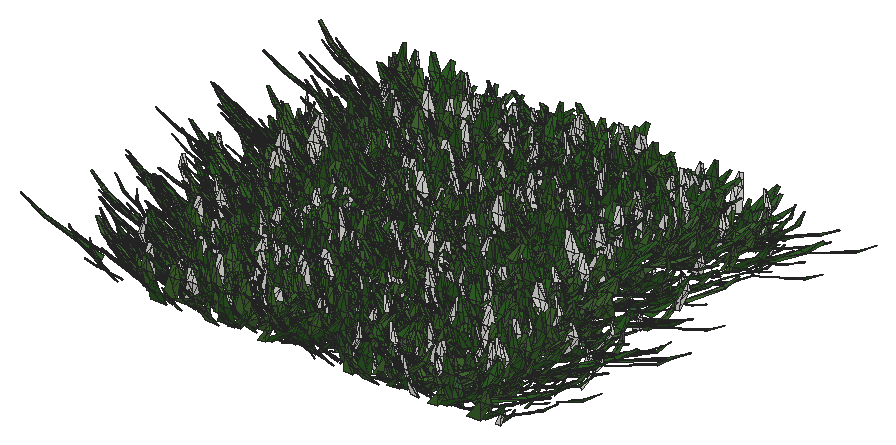
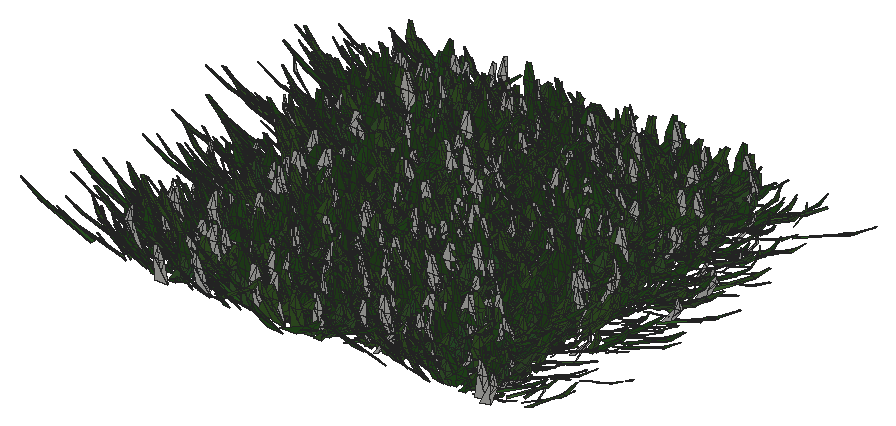
# SketchUp Ruby script. Lengths in inches.
U = 1.inch
M = Sketchup.active_model
def pt(a) = Geom::Point3d.new(a.map { |v| v * U })
def face(e, loops, mat)
  f = e.add_face(loops[0].map { |a| pt(a) })
  loops[1..].each { |l| e.add_face(l.map { |a| pt(a) }).erase! }
  f.material = f.back_material = mat if mat
  f
end
# faces: each face lists its corners as indices into pts; further lists are holes
def faces(e, pts, list, mat = nil) = list.each { |f| face(e, (f[0].is_a?(Array) ? f : [f]).map { |l| l.map { |i| pts[i] } }, mat) }
# xy, xz, yz: faces in a plane at the given z, y or x. An outline is a flat list of corners, or four numbers for a rectangle; further outlines are holes
def ring(l) = l.size == 4 ? [[l[0], l[1]], [l[2], l[1]], [l[2], l[3]], [l[0], l[3]]] : l.each_slice(2).to_a
def flat(e, list, mat, &to3) = list.each { |f| face(e, (f[0].is_a?(Array) ? f : [f]).map { |l| ring(l).map { |u, v| to3.(u, v) } }, mat) }
def xy(e, z, list, mat = nil) = flat(e, list, mat) { |x, y| [x, y, z] }
def xz(e, y, list, mat = nil) = flat(e, list, mat) { |x, z| [x, y, z] }
def yz(e, x, list, mat = nil) = flat(e, list, mat) { |y, z| [x, y, z] }
def lines(e, pts, list) = list.each { |a, b| e.add_line(pt(pts[a]), pt(pts[b])) }
# prism: a flat outline (further loops are holes) pulled along v
def prism(e, loops, v, mat = nil)
  f = face(e, loops, mat); d = Geom::Vector3d.new(v.map { |x| x * U })
  f.pushpull(f.normal.samedirection?(d) ? d.length : -d.length)
end
def box(e, o, s, mat = nil) = prism(e, [[o, [o[0] + s[0], o[1], o[2]], [o[0] + s[0], o[1] + s[1], o[2]], [o[0], o[1] + s[1], o[2]]]], [0, 0, s[2]], mat)
def at(x, y, z, deg = 0) = Geom::Transformation.translation(pt([x, y, z])) * Geom::Transformation.rotation(ORIGIN, Z_AXIS, deg.degrees)
def axes(o, x, y, z) = Geom::Transformation.new([*x, 0, *y, 0, *z, 0, *pt(o).to_a, 1])
def part(name) = M.definitions.add(name)
# library, detail: a bought-in or finely detailed component or shape, given as its bounding box
def library(name, o, s) = part(name).tap { |d| box(d.entities, o, s) }
def detail(e, o, s) = box(e.add_group.entities, o, s)
def put(e, d, t, mat = nil) = e.add_instance(d, t).tap { |i| i.material = mat if mat }
def group(e, t, mat = nil) = e.add_group.tap { |g| g.transformation = t; g.material = mat if mat }.entities
root = M.entities
M.materials.add("Material10").color = [48, 100, 38]
M.materials.add("Material3").color = [68, 110, 58]
M.materials.add("Material4").color = [48, 90, 38]
M.materials.add("Material5").color = [68, 110, 48]
M.materials.add("Material6").color = [48, 90, 48]
M.materials.add("Material7").color = [58, 110, 58]
M.materials.add("Material8").color = [58, 90, 38]
M.materials.add("Material9").color = [68, 100, 58]
c1 = part("grass00")
p = [[-0.6875,0.15,0],[-0.56,0.08,5.52],[-0.04,0.03,2.76],[0.48,-0.02,0],[0.35,-0.02,5.52],[-0.1,-0.14,5.52],
  [-0.12,0.65,8.37],[-0.42,0.65,8.37]]
faces(c1.entities,p,[[0,1,2,3],[3,2,4],[1,5,2],[5,4,2],[1,6,5],[4,5,6],[7,6,1]])
c2 = part("Group16\#1")
put(c2.entities,c1,axes([1.44,-0.61,-0.01],[0.05352,0.12609,0],[-0.10704,0.04543,0.07239],[0.06664,-0.02828,0.11628]),"Material6")
put(c2.entities,c1,axes([0.76,-0.15,-0.01],[0.04676,0.24062,0],[-0.23162,0.04501,0.06642],[0.0652,-0.01267,0.23595]),"Material3")
put(c2.entities,c1,axes([0.79,0.01,-0.01],[-0.00606,0.34651,0],[-0.34381,-0.00602,0.0432],[0.04319,0.00076,0.34386]))
put(c2.entities,c1,axes([1,0.23,-0.01],[-0.07192,0.31144,0],[-0.28722,-0.06632,0.1236],[0.12043,0.02781,0.29478]),"Material5")
put(c2.entities,c1,axes([1.66,0.77,-0.01],[-0.13828,0.29651,0],[-0.21551,-0.1005,0.22471],[0.20365,0.09498,0.23779]),"Material10")
put(c2.entities,c1,axes([0.6875,0.52,-0.01],[-0.18126,0.24051,0],[-0.22746,-0.17142,0.09788],[0.07817,0.05891,0.28481]),"Material5")
put(c2.entities,c1,axes([0.68,0.78,-0.01],[-0.215,0.18688,0],[-0.12385,-0.14248,0.21334],[0.13995,0.16101,0.18878]),"Material3")
put(c2.entities,c1,axes([0.56,1,-0.01],[-0.13756,0.07624,0],[-0.06159,-0.11112,0.0927],[0.04494,0.08108,0.12705]),"Material5")
put(c2.entities,c1,axes([0.2,0.64,-0.01],[-0.23729,0.07254,0],[-0.05711,-0.18681,0.153],[0.04473,0.14632,0.19535]),"Material10")
put(c2.entities,c1,axes([0.0625,0.72,-0.01],[-0.28874,0.02525,0],[-0.02179,-0.24916,0.14647],[0.01276,0.14591,0.25012]),"Material3")
put(c2.entities,c1,axes([-0.08,0.62,-0.01],[-0.34089,-0.04187,0],[0.03255,-0.26504,0.216],[-0.02633,0.21439,0.26703]),"Material10")
put(c2.entities,c1,axes([-0.34,0.98,-0.01],[-0.14314,-0.0493,0],[0.04397,-0.12769,0.06843],[-0.02228,0.0647,0.13505]),"Material10")
put(c2.entities,c1,axes([-0.87,1.45,-0.01],[-0.23488,-0.14114,0],[0.13761,-0.22901,0.06087],[-0.03135,0.05217,0.26717]))
put(c2.entities,c1,axes([-0.72,0.77,-0.01],[-0.14208,-0.13251,0],[0.07209,-0.0773,0.16301],[-0.11118,0.11922,0.1057]),"Material10")
put(c2.entities,c1,axes([-0.62,0.43,-0.01],[-0.14845,-0.21203,0],[0.18654,-0.13061,0.12304],[-0.10079,0.07057,0.22772]),"Material3")
put(c2.entities,c1,axes([-0.68,0.29,-0.01],[-0.13639,-0.32136,0],[0.31723,-0.13464,0.05579],[-0.05136,0.0218,0.34462]),"Material4")
put(c2.entities,c1,axes([-0.64,0.125,-0.01],[-0.0458,-0.23569,0],[0.22124,-0.043,0.08276],[-0.08124,0.01579,0.22538]),"Material7")
put(c2.entities,c1,axes([-1.6,-0.03,-0.01],[0.00576,-0.32897,0],[0.27526,0.00482,0.18018],[-0.18015,-0.00315,0.2753]),"Material5")
put(c2.entities,c1,axes([-1.36,-0.31,-0.01],[0.05718,-0.24765,0],[0.18172,0.04196,0.17267],[-0.16825,-0.03885,0.1865]),"Material10")
put(c2.entities,c1,axes([-1.54,-0.72,-0.01],[0.06537,-0.14017,0],[0.13555,0.06321,0.03939],[-0.0357,-0.01665,0.14956]))
put(c2.entities,c1,axes([-1.19,-0.9,-0.01],[0.09597,-0.12735,0],[0.11214,0.08451,0.07557],[-0.06035,-0.04548,0.14042]),"Material9")
put(c2.entities,c1,axes([-0.47,-0.54,-0.01],[0.11588,-0.10072,0],[0.0618,0.0711,0.12124],[-0.07953,-0.0915,0.0942]))
put(c2.entities,c1,axes([-0.47,-0.84,-0.01],[0.11927,-0.0661,0],[0.06603,0.11913,0.00646],[-0.00313,-0.00565,0.13621]),"Material5")
put(c2.entities,c1,axes([-0.38,-1.24,-0.01],[0.28037,-0.08571,0],[0.0618,0.20215,0.20315],[-0.05939,-0.19428,0.21139]),"Material9")
put(c2.entities,c1,axes([-0.06,-0.66,-0.01],[0.22719,-0.01987,0],[0.01247,0.14255,0.17758],[-0.01547,-0.17691,0.1431]),"Material8")
put(c2.entities,c1,axes([0.11,-0.89,-0.01],[0.14882,0.01828,0],[-0.01058,0.08611,0.12229],[0.01491,-0.12138,0.08676]),"Material6")
put(c2.entities,c1,axes([0.25,-0.72,-0.01],[0.20481,0.07053,0],[-0.06206,0.18022,0.10291],[0.03351,-0.0973,0.1906]),"Material6")
put(c2.entities,c1,axes([0.85,-1.42,-0.01],[0.16481,0.09904,0],[-0.09472,0.15762,0.05616],[0.02893,-0.04814,0.18389]),"Material5")
put(c2.entities,c1,axes([1.01,-1.09,-0.01],[0.21858,0.20385,0],[-0.17495,0.1876,0.15339],[0.10462,-0.11218,0.25652]),"Material10")
put(c2.entities,c1,axes([1.01,-0.71,-0.01],[0.08733,0.12473,0],[-0.06445,0.04512,0.13037],[0.1068,-0.07477,0.07867]),"Material6")
c3 = part("Group15\#1")
put(c3.entities,c2,at(0,0,0))
c4 = part("3darcstudiotree_grass00\#1")
put(c4.entities,c3,at(0,0,0))
put(root,c4,axes([260.58,70.62,7.6],[-3.85189,-0.43073,0],[1.56903,-0.87695,-0.00732],[0.02092,-0.01169,1.68082]))
put(root,c4,axes([260.53,52.63,7.6],[-1.50152,-0.9142,0],[4.09435,-0.4203,-0.04381],[0.2556,-0.02624,1.74465]))
put(root,c4,axes([261.21,61.66,7.6],[-0.92252,-0.87304,0],[4.75689,-0.31416,-0.01354],[0.0811,-0.00536,1.90468]))
put(root,c4,axes([260.04,81.46,7.6],[4.15823,-0.14638,0],[0.56684,1.00637,-0.04526],[0.04452,0.07905,1.7925]))
put(root,c4,axes([261.71,44.78,7.6],[-1.25145,-1.20565,0],[3.82205,-0.24795,-0.03225],[0.20024,-0.01299,1.58326]))
put(root,c4,axes([261.0625,68.85,7.6],[-3.10495,0.65805,0],[-2.73218,-0.80572,-0.0209],[-0.07578,-0.02235,1.48072]))
put(root,c4,axes([260.32,58.03,7.6],[4.00072,0.7254,0],[-2.30793,0.79554,-0.01189],[-0.04272,0.01473,1.50367]))
put(root,c4,axes([261.33,68.04,7.6],[-2.74027,0.72148,0],[-3.68495,-0.87475,-0.01749],[-0.07151,-0.01698,1.7911]))
put(root,c4,axes([261.68,55.01,7.6],[-2.75544,0.79472,0],[-3.06036,-0.66317,-0.04719],[-0.18345,-0.03975,1.30223]))
put(root,c4,axes([262.4,78.05,7.6],[1.11217,-0.96649,0],[4.59277,0.33032,-0.0144],[0.08373,0.00602,1.80693]))
put(root,c4,axes([262.5,64.79,7.6],[-4.93169,0.08818,0],[-0.36054,-1.26027,-0.06114],[-0.024,-0.08388,1.73764]))
put(root,c4,axes([260.64,62.9,7.6],[3.76135,0.71254,0],[-2.83931,0.93675,-0.0181],[-0.05013,0.01654,1.34745]))
put(root,c4,axes([261.02,73.98,7.6],[0.92537,1.06658,0],[-3.52867,0.19134,-0.00976],[-0.0687,0.00373,1.62508]))
put(root,c4,axes([262.56,46.16,7.6],[-4.59841,0.23812,0],[-1.05246,-1.27026,-0.05761],[-0.06188,-0.07469,1.71741]))
put(root,c4,axes([261.68,60.4,7.6],[3.52248,-0.74116,0],[2.46477,0.73213,-0.04982],[0.1917,0.05694,1.4295]))
put(root,c4,axes([262.16,66.49,7.6],[-2.75303,1.02553,0],[-3.67007,-0.61577,-0.03945],[-0.19029,-0.03193,1.6047]))
put(root,c4,axes([263.26,48.38,7.6],[0.13208,-1.10378,0],[4.58182,0.03427,-0.01737],[0.09381,0.0007,1.54781]))
put(root,c4,axes([262.03,82.16,7.6],[3.94098,0.32291,0],[-1.45311,1.10842,-0.04711],[-0.07836,0.05977,1.55738]))
put(root,c4,axes([263.88,56.61,7.6],[-4.05461,-0.34542,0],[1.65205,-1.21201,-0.06303],[0.10229,-0.07504,1.61067]))
put(root,c4,axes([262.77,49.89,7.6],[-0.37634,1.08622,0],[-3.78806,-0.08203,-0.04948],[-0.29529,-0.00639,1.42361]))
put(root,c4,axes([262.29,53.74,7.6],[1.93194,0.81354,0],[-3.84457,0.57061,-0.05173],[-0.21974,0.03261,1.38038]))
put(root,c4,axes([263.66,79.34,7.6],[2.66553,-1.02305,0],[4.32772,0.70474,-0.04483],[0.19345,0.0315,1.66248]))
put(root,c4,axes([263.7,76.32,7.6],[-4.37352,0.6514,0],[-2.31701,-0.97227,-0.00882],[-0.02275,-0.00955,1.42641]))
put(root,c4,axes([263.11,50.94,7.6],[4.99102,-0.01521,0],[0.04604,0.94447,-0.04731],[0.00388,0.07956,1.58849]))
put(root,c4,axes([264.25,74.9,7.6],[3.89455,0.04164,0],[-0.19515,1.14083,-0.05798],[-0.01392,0.08139,1.60438]))
put(root,c4,axes([263.95,71.87,7.6],[2.5974,0.75785,0],[-3.87592,0.83025,-0.05975],[-0.19783,0.04238,1.3909]))
put(root,c4,axes([267.01,64.96,7.6],[-4.50466,-0.2627,0],[0.84333,-0.90382,-0.01564],[0.02098,-0.02248,1.3694]))
put(root,c4,axes([267.65,61.36,7.6],[-4.10148,-0.37644,0],[1.4137,-0.96268,-0.02574],[0.04791,-0.03263,1.38465]))
put(root,c4,axes([267.53,58.8,7.6],[-4.28392,0.00118,0],[-0.00439,-0.99985,-0.04481],[-0.00034,-0.07634,1.70362]))
put(root,c4,axes([267.77,73.27,7.6],[-4.02766,-0.18324,0],[0.7232,-0.9935,-0.02729],[0.03622,-0.04975,1.8715]))
put(root,c4,axes([267.625,75.55,7.6],[1.16692,-1.18724,0],[4.2577,0.26155,-0.05295],[0.37072,0.02277,1.97565]))
put(root,c4,axes([268.55,69.08,7.6],[-4.78558,-0.30533,0],[0.89073,-0.87254,-0.00096],[0.00166,-0.00163,1.58162]))
put(root,c4,axes([268.12,72.38,7.6],[1.62332,-1.0011,0],[4.766,0.48301,-0.03495],[0.18538,0.01879,1.83937]))
put(root,c4,axes([268.83,51.01,7.6],[-4.37321,-0.34262,0],[1.17174,-0.93477,-0.00157],[0.00264,-0.00211,1.37913]))
put(root,c4,axes([268.33,70.08,7.6],[0.5215,-1.25098,0],[3.70627,0.09657,-0.02929],[0.19507,0.00508,1.55926]))
put(root,c4,axes([268.77,45.28,7.6],[-1.52927,-0.99373,0],[4.10162,-0.3945,-0.0371],[0.24735,-0.02379,1.96201]))
put(root,c4,axes([268.54,80.24,7.6],[-2.5925,0.65112,0],[-2.57682,-0.64124,-0.04592],[-0.2048,-0.05096,1.42994]))
put(root,c4,axes([267.57,62.73,7.6],[2.46517,0.89808,0],[-3.36918,0.57801,-0.0512],[-0.22975,0.03942,1.38975]))
put(root,c4,axes([268.32,56.94,7.6],[-1.95791,0.95694,0],[-3.80128,-0.48609,-0.05082],[-0.22925,-0.02932,1.35221]))
put(root,c4,axes([267.53,55.75,7.6],[3.4935,0.9356,0],[-3.37227,0.78699,-0.04297],[-0.21601,0.05041,1.98261]))
put(root,c4,axes([269.14,59.51,7.6],[-3.83195,0.74101,0],[-2.84787,-0.92045,-0.05181],[-0.15821,-0.05114,1.45196]))
put(root,c4,axes([269.32,78.68,7.6],[1.45199,-1.1226,0],[3.82197,0.30896,-0.02554],[0.13596,0.01099,1.40467]))
put(root,c4,axes([269.21,68.02,7.6],[0.21484,-1.19151,0],[3.62833,0.04089,-0.03915],[0.33615,0.00379,1.95085]))
put(root,c4,axes([269.36,54.43,7.6],[-4.05301,0.5506,0],[-2.43371,-1.11967,-0.04664],[-0.11424,-0.05256,1.63424]))
put(root,c4,axes([269.22,66.53,7.6],[2.22271,-0.98365,0],[3.97274,0.56106,-0.05349],[0.32137,0.04539,1.96798]))
put(root,c4,axes([268.12,81.1,7.6],[2.83397,0.77998,0],[-3.02687,0.68736,-0.01914],[-0.0787,0.01787,1.41957]))
put(root,c4,axes([267.94,46.38,7.6],[1.59207,1.04289,0],[-4.49774,0.42914,-0.00597],[-0.03376,0.00322,1.82255]))
put(root,c4,axes([268.57,43.8,7.6],[3.98575,0.27966,0],[-0.97946,0.87245,-0.00495],[-0.0082,0.00731,1.38942]))
put(root,c4,axes([268.85,76.19,7.6],[4.21135,-0.01817,0],[0.08044,1.16521,-0.0287],[0.00337,0.04884,1.98369]))
put(root,c4,axes([269.33,49.39,7.6],[-2.028,0.74895,0],[-3.60661,-0.61038,-0.00267],[-0.01315,-0.00223,1.62102]))
put(root,c4,axes([270.14,52.07,7.6],[3.07423,-0.81379,0],[3.32943,0.78609,-0.05261],[0.18555,0.04381,1.38839]))
put(root,c4,axes([269.4,47.71,7.6],[3.5941,0.56914,0],[-2.69156,1.06232,-0.01012],[-0.02733,0.01079,1.58691]))
put(root,c4,axes([272.29,50.95,7.6],[-0.91152,-0.89442,0],[3.63132,-0.23129,-0.03395],[0.21582,-0.01375,1.53644]))
put(root,c4,axes([272.67,53.47,7.6],[-0.47866,-0.98426,0],[5.08014,-0.15441,-0.04217],[0.1851,-0.00563,1.41426]))
put(root,c4,axes([272.86,64.8125,7.6],[-3.99249,-0.2843,0],[1.19862,-1.05202,-0.03955],[0.07734,-0.06788,1.95202]))
put(root,c4,axes([272.04,57.35,7.6],[4.25304,-0.27501,0],[1.24647,1.20478,-0.04841],[0.06924,0.06692,1.77682]))
put(root,c4,axes([272.32,69,7.6],[3.55406,-0.41539,0],[2.08359,1.1142,-0.04906],[0.12364,0.06612,1.82977]))
put(root,c4,axes([273.625,46.28,7.6],[-0.93715,-1.08339,0],[4.95712,-0.268,-0.05631],[0.2396,-0.01295,1.37991]))
put(root,c4,axes([273.91,55.33,7.6],[-3.14134,-0.50366,0],[2.13341,-0.83163,-0.01822],[0.06361,-0.0248,1.59761]))
put(root,c4,axes([273.65,48.91,7.6],[-3.94175,0.51659,0],[-1.67373,-0.7982,-0.02232],[-0.07314,-0.03488,1.59039]))
put(root,c4,axes([272.15,58.73,7.6],[1.62757,0.88807,0],[-4.34169,0.49732,-0.00338],[-0.01586,0.00182,1.53978]))
put(root,c4,axes([272.95,78.29,7.6],[4.57989,-0.16103,0],[0.69599,1.23718,-0.01318],[0.01167,0.02075,1.98636]))
put(root,c4,axes([274.32,61.36,7.6],[1.79397,-1.16047,0],[4.15779,0.40172,-0.011],[0.05477,0.00529,1.48653]))
put(root,c4,axes([274.81,45.33,7.6],[-3.09464,-0.54466,0],[2.39537,-0.85062,-0.03828],[0.16794,-0.05964,1.98208]))
put(root,c4,axes([273.47,67.29,7.6],[0.16957,1.15455,0],[-4.45398,0.04088,-0.05084],[-0.31058,0.00285,1.70302]))
put(root,c4,axes([273.97,71.875,7.6],[3.46351,-0.6215,0],[2.10035,0.73155,-0.02763],[0.09487,0.03304,1.3256]))
put(root,c4,axes([275.05,66.46,7.6],[-1.3865,-0.85758,0],[4.31936,-0.43646,-0.05241],[0.27908,-0.0282,1.67241]))
put(root,c4,axes([275.22,75.41,7.6],[-4.39937,-0.11992,0],[0.44419,-1.01847,-0.05296],[0.03633,-0.08329,1.62079]))
put(root,c4,axes([275.91,48.37,7.6],[-1.76031,-0.79386,0],[4.32977,-0.60005,-0.00731],[0.04086,-0.00566,1.97847]))
put(root,c4,axes([275.91,79.52,7.6],[-2.83446,-0.91757,0],[3.42874,-0.66198,-0.00917],[0.043,-0.0083,1.60374]))
put(root,c4,axes([275.57,73.66,7.6],[-0.96511,-1.1714,0],[4.02104,-0.20706,-0.02826],[0.17189,-0.00885,1.59374]))
put(root,c4,axes([274.75,76.5,7.6],[-2.51846,0.95711,0],[-4.14801,-0.68217,-0.04701],[-0.20561,-0.03381,1.62457]))
put(root,c4,axes([275.9375,60.11,7.6],[-3.64421,0.19897,0],[-0.82865,-0.94858,-0.01018],[-0.01217,-0.01393,1.35975]))
put(root,c4,axes([274.87,51.98,7.6],[4.36646,0.14498,0],[-0.67462,1.26988,-0.05242],[-0.04036,0.07596,1.87281]))
put(root,c4,axes([275.83,81.52,7.6],[3.61828,-0.3087,0],[1.22458,0.89709,-0.02189],[0.0555,0.04066,1.86062]))
put(root,c4,axes([275.97,62.55,7.6],[-0.33218,0.92371,0],[-3.73108,-0.08386,-0.0349],[-0.21038,-0.00473,1.41691]))
put(root,c4,axes([276.03,71.04,7.6],[3.6543,-0.06929,0],[0.34871,1.14948,-0.06006],[0.02412,0.07952,1.53056]))
put(root,c4,axes([276.53,82.52,7.6],[2.4776,1.07425,0],[-3.76626,0.5429,-0.02249],[-0.11657,0.0168,1.62577]))
put(root,c4,axes([278.52,70.97,7.6],[1.28704,-1.14477,0],[4.41434,0.31018,-0.04021],[0.23445,0.01647,1.73573]))
put(root,c4,axes([278.91,76.45,7.6],[-3.66743,0.44114,0],[-1.9663,-1.02167,-0.05656],[-0.13362,-0.06943,1.54444]))
put(root,c4,axes([279.11,81.31,7.6],[-3.63818,0.44085,0],[-1.59896,-0.82474,-0.04774],[-0.15109,-0.07793,1.66266]))
put(root,c4,axes([279.53,46.66,7.6],[-3.07397,-0.63014,0],[2.5257,-0.77005,-0.04795],[0.16981,-0.05177,1.39039]))
put(root,c4,axes([278.5,48.86,7.6],[3.59272,-0.42375,0],[1.98946,1.05421,-0.02435],[0.06043,0.03202,1.69455]))
put(root,c4,axes([279.69,74.86,7.6],[-2.26382,-1.02381,0],[3.25832,-0.45029,-0.04183],[0.23401,-0.03234,1.48723]))
put(root,c4,axes([279.79,59.42,7.6],[-1.57651,-1.12747,0],[4.0703,-0.35571,-0.03865],[0.26242,-0.02293,1.9383]))
put(root,c4,axes([278.36,73.07,7.6],[1.17301,1.14331,0],[-4.44463,0.28501,-0.04684],[-0.2246,0.0144,1.41954]))
put(root,c4,axes([278.55,65.09,7.6],[4.31123,0.22817,0],[-0.83721,0.9887,-0.03259],[-0.04316,0.05097,1.61556]))
put(root,c4,axes([278.54,79.93,7.6],[3.06774,1.03902,0],[-3.08129,0.5686,-0.03251],[-0.17928,0.03308,1.64081]))
put(root,c4,axes([280.92,72.3125,7.6],[-2.08621,-0.85991,0],[3.58173,-0.54309,-0.01057],[0.06396,-0.0097,1.85267]))
put(root,c4,axes([280.55,61.49,7.6],[-4.18093,0.10999,0],[-0.54376,-1.29184,-0.00853],[-0.00476,-0.01131,1.7318]))
put(root,c4,axes([281.32,51.4,7.6],[-3.42299,-0.52038,0],[2.6642,-1.0953,-0.06276],[0.1523,-0.06261,1.49667]))
put(root,c4,axes([279.54,48.14,7.6],[3.25907,0.53746,0],[-2.27195,0.86105,-0.03997],[-0.15705,0.05952,1.84008]))
put(root,c4,axes([281.5625,53.51,7.6],[-2.53551,-0.66282,0],[3.06498,-0.73279,-0.03327],[0.11879,-0.0284,1.30962]))
put(root,c4,axes([280.36,69.43,7.6],[-1.21767,0.90066,0],[-3.71776,-0.31415,-0.04196],[-0.263,-0.02222,1.62262]))
put(root,c4,axes([281.64,56.78,7.6],[-4.32463,-0.20055,0],[0.81802,-1.10246,-0.00704],[0.00853,-0.0115,1.86241]))
put(root,c4,axes([280.12,65.59,7.6],[-0.94156,1.16657,0],[-3.85079,-0.19425,-0.00527],[-0.04036,-0.00204,1.91768]))
put(root,c4,axes([280.44,63.23,7.6],[-1.89095,0.77708,0],[-4.00997,-0.60986,-0.02284],[-0.10942,-0.01664,1.64481]))
put(root,c4,axes([281.24,77.73,7.6],[-3.52622,0.53949,0],[-2.34194,-0.95671,-0.04749],[-0.11586,-0.04733,1.3106]))
put(root,c4,axes([280.89,51.9,7.6],[-0.72165,1.07172,0],[-4.22626,-0.17786,-0.04712],[-0.23093,-0.00972,1.33133]))
put(root,c4,axes([280.45,55.59,7.6],[1.97727,0.77994,0],[-4.30152,0.68157,-0.01772],[-0.06482,0.01027,1.37883]))
put(root,c4,axes([281.86,44.85,7.6],[3.9848,-0.55599,0],[2.03989,0.91374,-0.03495],[0.12387,0.05549,1.90256]))
put(root,c4,axes([281.67,82.29,7.6],[-0.75919,1.1846,0],[-4.72482,-0.18925,-0.01053],[-0.05452,-0.00218,1.56894]))
put(root,c4,axes([282.44,58.02,7.6],[-2.69032,0.86465,0],[-3.81847,-0.74256,-0.01031],[-0.04487,-0.00873,1.66779]))
put(root,c4,axes([281.81,67.3,7.6],[4.37586,0.6715,0],[-2.05906,0.83863,-0.0354],[-0.14622,0.05955,1.94218]))
put(root,c4,axes([284.52,81.49,7.6],[3.53194,-0.86434,0],[3.34252,0.85365,-0.00616],[0.02391,0.00611,1.65812]))
put(root,c4,axes([284.12,52.5,7.6],[-1.22084,1.17012,0],[-4.22614,-0.27558,-0.04083],[-0.27889,-0.01819,1.92702]))
put(root,c4,axes([285.35,66.53,7.6],[2.5391,-0.86121,0],[4.09888,0.75529,-0.00987],[0.04755,0.00876,1.9048]))
put(root,c4,axes([284.69,62.82,7.6],[4.20042,-0.44882,0],[1.64886,0.96446,-0.01454],[0.02841,0.01662,1.30369]))
put(root,c4,axes([285.74,77,7.6],[-3.69839,0.06543,0],[-0.3293,-1.16339,-0.01026],[-0.00422,-0.01493,1.70108]))
put(root,c4,axes([285.24,72.49,7.6],[2.45158,-0.94892,0],[4.05066,0.65407,-0.0579],[0.29835,0.04817,1.84885]))
put(root,c4,axes([285.61,61.375,7.6],[-3.62062,0.56511,0],[-2.64905,-1.06077,-0.02972],[-0.08176,-0.03274,1.62371]))
put(root,c4,axes([284.95,70.45,7.6],[4.94305,-0.26827,0],[1.01972,1.17431,-0.03342],[0.04517,0.05201,1.91382]))
put(root,c4,axes([285.51,44.5,7.6],[5.06338,0.28931,0],[-0.91613,1.00212,-0.00333],[-0.00395,0.00432,1.36941]))
put(root,c4,axes([287.32,49.57,7.6],[-3.99538,-0.04123,0],[0.20618,-1.24865,-0.05407],[0.01202,-0.0728,1.68402]))
put(root,c4,axes([285.74,46.04,7.6],[2.5961,0.65731,0],[-3.59247,0.8868,-0.04002],[-0.16483,0.04069,1.82631]))
put(root,c4,axes([286.79,59.92,7.6],[-3.34956,0.74843,0],[-3.0511,-0.85344,-0.02716],[-0.08391,-0.02347,1.32671]))
put(root,c4,axes([288.02,58.25,7.6],[-2.33326,-1.15563,0],[4.19034,-0.52878,-0.02075],[0.1057,-0.01334,1.67433]))
put(root,c4,axes([286.73,77.81,7.6],[3.85684,-0.72833,0],[2.27457,0.7528,-0.01203],[0.05895,0.01951,1.91781]))
put(root,c4,axes([287.96,50.96,7.6],[-4.81633,-0.15482,0],[0.50253,-0.97708,-0.03967],[0.03663,-0.07121,1.78282]))
put(root,c4,axes([287.84,69.46,7.6],[-4.3189,0.23802,0],[-0.87038,-0.98708,-0.01188],[-0.02021,-0.02292,1.99665]))
put(root,c4,axes([287.27,64.42,7.6],[3.261,-0.91173,0],[3.2122,0.71807,-0.03435],[0.17461,0.03903,1.83666]))
put(root,c4,axes([286.56,73.68,7.6],[0.9409,1.10722,0],[-4.02636,0.21385,-0.01067],[-0.07425,0.00394,1.82972]))
put(root,c4,axes([288.29,55.74,7.6],[-4.23033,0.08475,0],[-0.4056,-1.2654,-0.02116],[-0.00955,-0.02979,1.79229]))
put(root,c4,axes([287.84,74.71,7.6],[3.52347,0.24028,0],[-1.10282,1.01075,-0.00322],[-0.00644,0.0059,1.99197]))
put(root,c4,axes([287.73,67.09,7.6],[1.43969,0.92574,0],[-4.67724,0.45462,-0.01993],[-0.11798,0.01147,1.99239]))
put(root,c4,axes([288.37,57.28,7.6],[5.05994,-0.2516,0],[1.00622,1.26478,-0.02703],[0.02801,0.03521,1.71263]))
put(root,c4,axes([288.25,53.36,7.6],[4.82559,0.20741,0],[-0.80452,1.16986,-0.00744],[-0.0078,0.01134,1.83611]))
put(root,c4,axes([288.52,79.36,7.6],[0.8534,1.21084,0],[-4.69984,0.20703,-0.04576],[-0.24908,0.01097,1.64855]))
put(root,c4,axes([288.34,47.93,7.6],[3.19918,0.93159,0],[-3.22991,0.69324,-0.03135],[-0.15607,0.0335,1.74596]))
put(root,c4,axes([290.27,58.24,7.6],[-4.78772,-0.06379,0],[0.24177,-1.13418,-0.04256],[0.01334,-0.06257,1.67228]))
put(root,c4,axes([290.96,52.52,7.6],[-0.71675,-1.13994,0],[5.03401,-0.19782,-0.0381],[0.22843,-0.00898,1.93318]))
put(root,c4,axes([290.88,69.1,7.6],[-3.55446,-0.53666,0],[1.86548,-0.77223,-0.04514],[0.17034,-0.07051,1.64638]))
put(root,c4,axes([290.88,74.66,7.6],[-3.57017,-0.151,0],[0.63334,-0.9359,-0.02254],[0.02209,-0.03264,1.39425]))
put(root,c4,axes([290.3,49.03,7.6],[3.4593,-0.56145,0],[2.1047,0.8105,-0.02789],[0.10781,0.04152,1.71527]))
put(root,c4,axes([291.21,50.41,7.6],[-3.94355,0.22015,0],[-0.99731,-1.11654,-0.00123],[-0.00186,-0.00209,1.99006]))
put(root,c4,axes([290.75,78.17,7.6],[3.30228,-0.99674,0],[2.91611,0.60383,-0.04892],[0.25342,0.05247,1.59182]))
put(root,c4,axes([290.27,77.02,7.6],[4.61986,0.38616,0],[-1.27131,0.9506,-0.01696],[-0.03888,0.02907,1.81122]))
put(root,c4,axes([291.47,81.05,7.6],[-2.0103,0.88344,0],[-3.56839,-0.5075,-0.04597],[-0.20616,-0.02932,1.32398]))
put(root,c4,axes([291.27,82.59,7.6],[3.96671,-0.47551,0],[1.66213,0.8666,-0.03326],[0.09836,0.05128,1.64345]))
put(root,c4,axes([291.07,47.7,7.6],[2.08308,0.83791,0],[-3.29361,0.51175,-0.00184],[-0.01033,0.00161,1.60144]))
put(root,c4,axes([291.53,64.84,7.6],[-1.06068,0.91839,0],[-4.56893,-0.3298,-0.01983],[-0.09265,-0.00669,1.44555]))
put(root,c4,axes([292.07,44.94,7.6],[-1.97754,0.85348,0],[-3.2966,-0.47739,-0.02138],[-0.12695,-0.01838,1.63406]))
put(root,c4,axes([292.0625,57.29,7.6],[-1.2265,1.05965,0],[-4.78236,-0.34596,-0.06381],[-0.32881,-0.02379,1.66913]))
